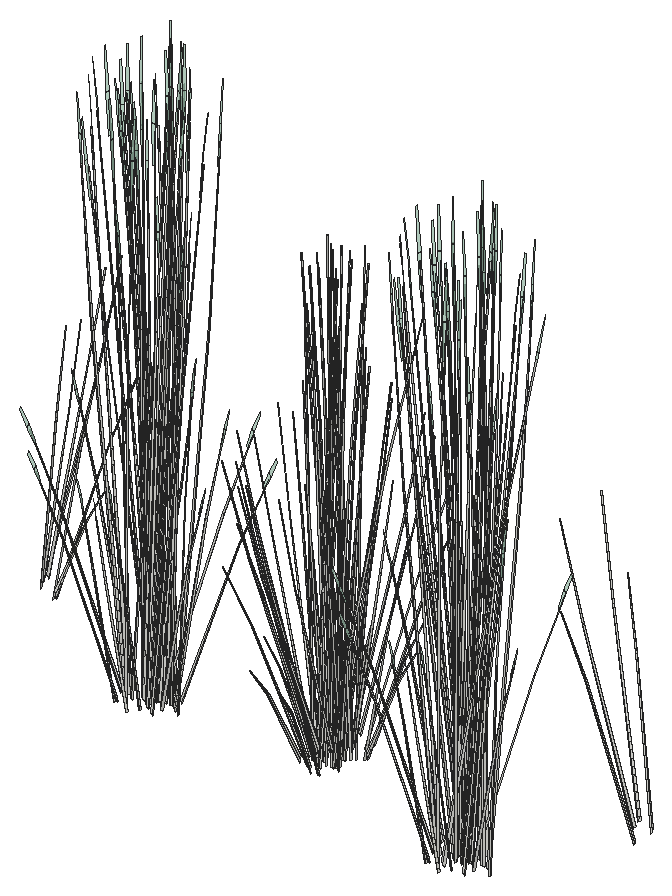
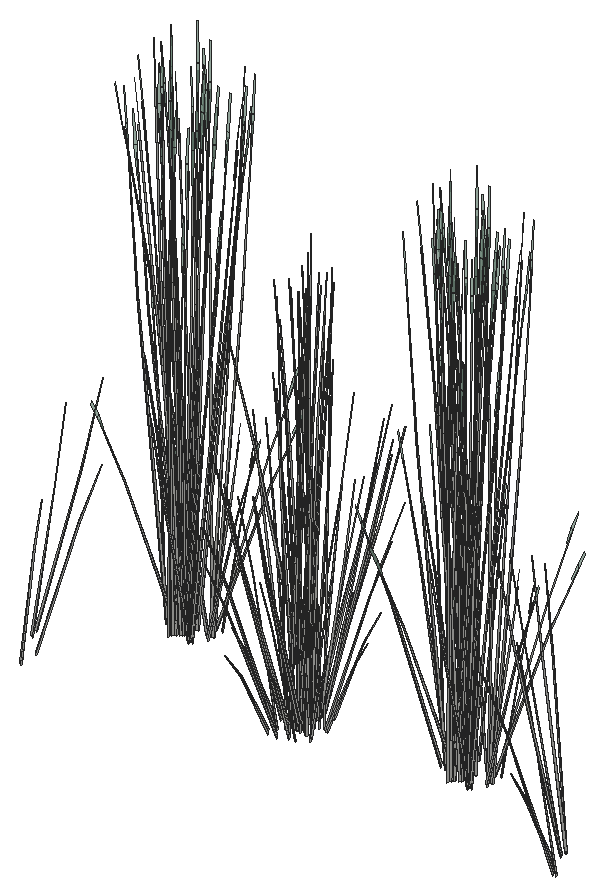
# SketchUp Ruby script. Lengths in inches.
U = 1.inch
M = Sketchup.active_model
def pt(a) = Geom::Point3d.new(a.map { |v| v * U })
def face(e, loops, mat)
  f = e.add_face(loops[0].map { |a| pt(a) })
  loops[1..].each { |l| e.add_face(l.map { |a| pt(a) }).erase! }
  f.material = f.back_material = mat if mat
  f
end
# faces: each face lists its corners as indices into pts; further lists are holes
def faces(e, pts, list, mat = nil) = list.each { |f| face(e, (f[0].is_a?(Array) ? f : [f]).map { |l| l.map { |i| pts[i] } }, mat) }
# xy, xz, yz: faces in a plane at the given z, y or x. An outline is a flat list of corners, or four numbers for a rectangle; further outlines are holes
def ring(l) = l.size == 4 ? [[l[0], l[1]], [l[2], l[1]], [l[2], l[3]], [l[0], l[3]]] : l.each_slice(2).to_a
def flat(e, list, mat, &to3) = list.each { |f| face(e, (f[0].is_a?(Array) ? f : [f]).map { |l| ring(l).map { |u, v| to3.(u, v) } }, mat) }
def xy(e, z, list, mat = nil) = flat(e, list, mat) { |x, y| [x, y, z] }
def xz(e, y, list, mat = nil) = flat(e, list, mat) { |x, z| [x, y, z] }
def yz(e, x, list, mat = nil) = flat(e, list, mat) { |y, z| [x, y, z] }
def lines(e, pts, list) = list.each { |a, b| e.add_line(pt(pts[a]), pt(pts[b])) }
# prism: a flat outline (further loops are holes) pulled along v
def prism(e, loops, v, mat = nil)
  f = face(e, loops, mat); d = Geom::Vector3d.new(v.map { |x| x * U })
  f.pushpull(f.normal.samedirection?(d) ? d.length : -d.length)
end
def box(e, o, s, mat = nil) = prism(e, [[o, [o[0] + s[0], o[1], o[2]], [o[0] + s[0], o[1] + s[1], o[2]], [o[0], o[1] + s[1], o[2]]]], [0, 0, s[2]], mat)
def at(x, y, z, deg = 0) = Geom::Transformation.translation(pt([x, y, z])) * Geom::Transformation.rotation(ORIGIN, Z_AXIS, deg.degrees)
def axes(o, x, y, z) = Geom::Transformation.new([*x, 0, *y, 0, *z, 0, *pt(o).to_a, 1])
def part(name) = M.definitions.add(name)
# library, detail: a bought-in or finely detailed component or shape, given as its bounding box
def library(name, o, s) = part(name).tap { |d| box(d.entities, o, s) }
def detail(e, o, s) = box(e.add_group.entities, o, s)
def put(e, d, t, mat = nil) = e.add_instance(d, t).tap { |i| i.material = mat if mat }
def group(e, t, mat = nil) = e.add_group.tap { |g| g.transformation = t; g.material = mat if mat }.entities
root = M.entities
M.materials.add("LightPink_Translucent").color = [175, 214, 192]
M.materials["LightPink_Translucent"].alpha = 0.75
c1 = part("blade")
p = [[2.15,0.21,22],[0,0.17,0],[0.09,0.45,0],[2.18,0.31,22],[2.29,0.31,22],[0.38,0.45,0],
  [2.48,0.24,33],[2.49,0.24,33],[2.48,0.22,33]]
faces(c1.entities,p,[[0,1,2,3],[4,5,2,3],[6,3,4,7],[8,0,3,6]])
c2 = part("blade with seeds\#1")
put(c2.entities,c1,at(0,0,0))
c3 = part("seeds")
p = [[0.3,-0.1,1.38],[-0.01,-0.03,1.59],[-0.01,-0.03,0.03],[0.14,-0.07,-0.07],[0.29,-0.03,3],[0.15,0.01,3.11]]
faces(c3.entities,p,[[0,1,2,3],[1,0,4,5]],"LightPink_Translucent")
c4 = part("blade with seeds")
put(c4.entities,c1,at(0,0,0))
put(c4.entities,c3,axes([2.4,0.25,30.99],[1.5799,-0.05474,1.17369],[-0.12525,1.92788,0.29478],[-0.07173,-0.02425,1.56792]))
put(root,c2,axes([413.42,244.55,138.99],[-0.22657,0.01287,0.94226],[0.1616,-0.32149,0.69231],[0.10799,0.06323,0.20754]))
put(root,c2,axes([412.55,244.43,140.82],[0.25603,-0.35588,-0.4653],[0.22422,0.37594,-0.36041],[0.13008,0.05415,0.89031]))
put(root,c2,axes([412.8,243.375,140.56],[0.09552,-0.48869,-0.41919],[0.3275,0.16751,-0.3247],[0.13186,-0.04481,0.80208]))
put(root,c2,axes([412.93,244.82,139.03],[-0.06748,-0.45162,0.05338],[0.27185,-0.10383,-0.708],[0.13761,0.02863,0.63462]))
put(root,c2,axes([412.43,244.54,141.1],[0.35246,0.01294,-0.64693],[-0.02367,0.54471,0.07807],[0.14932,0.05748,0.91515]))
put(root,c2,axes([412.73,243.55,140.8],[0.30983,-0.23727,-0.58282],[0.17267,0.48842,0.07033],[0.1497,-0.05548,0.82446]))
put(root,c2,axes([413.22,244.93,138.84],[-0.06011,-0.15688,1.17311],[0.18125,-0.38733,-0.25229],[0.15683,0.11528,0.50157]))
put(root,c4,axes([426.42,237.2,139.53],[0.1661,0.03656,1.30132],[0.10705,0.37341,-0.27986],[-0.22562,0.0699,0.55638]))
put(root,c4,axes([427.06,235.39,139.53],[0.09331,0.12399,1.30132],[-0.21502,0.33702,-0.27986],[-0.22079,-0.08055,0.55638]))
put(root,c4,axes([427.94,237.98,139.33],[-0.29882,0.44625,0],[-0.49993,-0.24886,-0.46963],[-0.11386,-0.05668,1.48977]))
put(root,c4,axes([427.4,238.63,139.53],[0.15082,-0.07025,1.30132],[0.37238,0.21183,-0.27986],[-0.11083,0.18329,0.55638]))
put(root,c4,axes([427.18,234.62,139.11],[-0.13787,0.36364,-0.03542],[-0.42434,-0.11186,-0.16061],[-0.06443,-0.05948,0.52975]))
put(root,c4,axes([427.82,234.16,139.53],[-0.02894,0.14568,1.30132],[-0.4231,0.12195,-0.27986],[-0.0989,-0.1883,0.55638]))
put(root,c4,axes([426.96,236.28,139.33],[-0.59763,0,0],[0,-0.49772,-0.46963],[0,-0.11336,1.48977]))
put(root,c4,axes([427.42,236.15,139.29],[-0.44456,0.37441,0.27988],[-0.44483,-0.37047,-0.33208],[-0.01552,-0.10632,1.50045]))
put(root,c4,axes([429.43,237.0625,139.41],[-0.4667,-0.35844,-0.22925],[0.39271,-0.40249,0.50168],[-0.12567,0.04193,1.53076]))
put(root,c4,axes([428.2,237.75,139.43],[0.44731,0.22267,0.45182],[-0.26736,0.39927,0],[-0.10188,-0.05071,1.43328]))
put(root,c4,axes([428.625,236.93,139.39],[0.12668,-0.5277,-0.2132],[0.60063,0.09198,0.46656],[-0.10495,-0.07287,1.42361]))
put(root,c4,axes([428.84,237.06,139.55],[-0.0922,0.39744,0.13176],[-0.45047,-0.06899,-0.37626],[-0.08198,-0.04081,1.15337]))
put(root,c4,axes([427.32,236.36,139.43],[0,0.44533,0.45182],[-0.53472,0,0],[0,-0.10143,1.43328]))
put(root,c4,axes([429.77,238.04,139.17],[-0.29509,-0.44781,-0.04679],[0.49993,-0.24886,0.46963],[-0.12319,0.04264,1.48904]))
put(root,c4,axes([427.5,238.29,139.74],[0.43418,-0.07886,0.05922],[0.09982,0.31771,-0.78537],[-0.02753,0.16083,0.70398]))
put(root,c4,axes([428.83,234.16,139.11],[-0.33028,0.25548,-0.03542],[-0.30262,-0.27981,-0.16061],[-0.02131,-0.07928,0.52975]))
put(root,c4,axes([428.69,236.68,139.32],[0.60408,0.09383,0.41637],[-0.12294,0.52992,0.16339],[-0.08828,-0.05117,1.44559]))
put(root,c4,axes([428.37,237.52,139.42],[0.51358,-0.1182,0.16054],[0.12682,0.43988,0.31929],[-0.0458,-0.06409,1.4597]))
put(root,c4,axes([429.03,237.59,139.17],[-0.48183,-0.19993,0],[0.23189,-0.41543,0],[0,0,1.48063]))
put(root,c4,axes([430.14,238.09,139.33],[0.29882,0.44625,0],[-0.49993,0.24886,-0.46963],[-0.11386,0.05668,1.48977]))
put(root,c4,axes([429.9,237.55,139.42],[0.13807,-0.44258,0.16054],[0.50524,0.12525,0.31929],[-0.08728,0.00216,1.4597]))
put(root,c4,axes([429.66,236.96,139.55],[0.3531,0.26757,0.13176],[-0.29453,0.30187,-0.37626],[-0.08198,0.04081,1.15337]))
put(root,c4,axes([429.54,236.63,139.26],[-0.44456,-0.3833,-0.05579],[0.44483,-0.38354,0],[-0.01552,-0.01339,1.5977]))
put(root,c4,axes([429.78,237.8125,139.29],[0.59835,0.14475,0.27988],[-0.14969,0.51739,-0.33208],[-0.09903,0.06475,1.50045]))
put(root,c4,axes([430.04,237.78,139.43],[0.44731,-0.22267,0.45182],[0.26736,0.39927,0],[-0.10188,0.05071,1.43328]))
put(root,c4,axes([428.64,236.1875,139.32],[0.2078,0.49797,0.41637],[-0.59373,0.17316,0.16339],[0.00726,-0.0915,1.44559]))
put(root,c4,axes([429.14,237.42,139.18],[-0.15594,-0.38394,0],[0.4453,-0.13445,0],[0,0,1.40478]))
put(root,c4,axes([430.69,236.42,139.42],[-0.37551,-0.32439,0.16054],[0.37842,-0.31463,0.31929],[-0.04147,0.06625,1.4597]))
put(root,c4,axes([429.39,236.23,139.18],[0,-0.51528,0],[0.59763,0,0],[0,0,1.63305]))
put(root,c4,axes([428.83,236.32,139.38],[0.53851,0.21584,0.21899],[-0.25917,0.44849,0.45502],[0,-0.10338,1.46094]))
put(root,c4,axes([429.6875,236.4375,139.26],[0,0.51503,-0.0513],[-0.59763,0,0],[0,0.01619,1.63225]))
put(root,c4,axes([428.42,235.24,139.42],[-0.13807,0.44258,0.16054],[-0.50524,-0.12525,0.31929],[0.08728,-0.00216,1.4597]))
put(root,c4,axes([429.4,237.43,139.25],[0.2078,0.51161,-0.05471],[-0.59373,0.17927,0],[0.00726,0.01787,1.56677]))
put(root,c4,axes([428.17,234.69,139.33],[-0.29882,-0.44625,0],[0.49993,-0.24886,-0.46963],[0.11386,-0.05668,1.48977]))
put(root,c4,axes([431.12,236.76,139.17],[-0.59734,-0.00356,-0.04529],[0,-0.49772,0.45448],[-0.01877,0.1133,1.441]))
put(root,c4,axes([429.95,235.26,139.42],[-0.51358,0.1182,0.16054],[-0.12682,-0.43988,0.31929],[0.0458,0.06409,1.4597]))
put(root,c4,axes([429.11,235.91,139.32],[-0.39628,0.40415,0.41637],[-0.4708,-0.35675,0.16339],[0.09554,-0.04033,1.44559]))
put(root,c4,axes([429.78,236.54,139.19],[0.33362,0.28765,0],[-0.33362,0.28765,0],[0,0,1.54032]))
put(root,c4,axes([429.58,237.6,139.18],[0.48183,0.19993,0],[-0.23189,0.41543,0],[0,0,1.59208]))
put(root,c4,axes([429.62,236.11,139.34],[-0.60408,-0.09383,0.44771],[0.12294,-0.52992,0.17569],[0.08828,0.05117,1.5544]))
put(root,c4,axes([429.79,236.35,139.18],[0.53472,0,0],[0,0.46104,0],[0,0,1.6235]))
put(root,c4,axes([429.98,236.3,139.55],[0.4453,-0.12987,0.13176],[0.15594,0.37086,-0.37626],[0,0.08162,1.15337]))
put(root,c4,axes([429.92,234.33,139.53],[-0.13585,0.09014,1.30132],[-0.40687,-0.15777,-0.27986],[0.07542,-0.19621,0.55638]))
put(root,c4,axes([430.99,236.43,139.43],[0,-0.44533,0.45182],[0.53472,0,0],[0,0.10143,1.43328]))
put(root,c4,axes([429.47,235.73,139.55],[0.0922,-0.39744,0.13176],[0.45047,0.06899,-0.37626],[0.08198,0.04081,1.15337]))
put(root,c4,axes([430.11,235.04,139.43],[-0.44731,-0.22267,0.45182],[0.26736,-0.39927,0],[0.10188,0.05071,1.43328]))
put(root,c4,axes([429.72,237.37,139.16],[0.50177,-0.1511,-0.1747],[0.17632,0.43526,0.00007],[0.05539,-0.0167,1.58246]))
put(root,c4,axes([429.59,237.63,139.53],[0.00843,-0.14762,1.30132],[0.40305,-0.1649,-0.27986],[0.12442,0.17669,0.55638]))
put(root,c4,axes([431.36,236.51,139.33],[0.59763,0,0],[0,0.49772,-0.46963],[0,0.11336,1.48977]))
put(root,c4,axes([430.37,234.81,139.33],[0.29882,-0.44625,0],[0.49993,0.24886,-0.46963],[0.11386,0.05668,1.48977]))
put(root,c4,axes([432.11,236.19,139.23],[-0.29631,-0.28477,-0.05904],[0.32453,-0.26092,-0.26768],[0.09195,-0.01837,0.88292]))
put(root,c4,axes([431.23,235.39,139.53],[-0.17074,-0.01319,1.30132],[-0.17492,-0.35385,-0.27986],[0.20976,-0.1001,0.55638]))
put(root,c4,axes([431.55,236.57,138.97],[-0.30783,0.05344,1.28841],[-0.049,-0.4254,0.07375],[0.2156,-0.06439,0.73315]))
put(root,c4,axes([431.63,237.2,139.53],[-0.1151,-0.10953,1.30132],[0.14976,-0.36232,-0.27986],[0.23288,0.04908,0.55638]))
put(root,c2,axes([443.83,237.48,138.9375],[0.07713,0.14131,1.17311],[-0.13499,0.4232,-0.25229],[-0.16789,-0.07845,0.50157]))
put(root,c2,axes([444.1,238.13,140.9],[-0.30983,0.23727,-0.58282],[-0.17267,-0.48842,0.07033],[-0.1497,0.05548,0.82446]))
put(root,c2,axes([443.6875,239.67,138.9375],[0.12465,0.0301,1.17311],[0.10435,0.44009,-0.25229],[-0.16111,0.10287,0.50157]))
put(root,c2,axes([444.41,237.14,140.9],[-0.35246,-0.01294,-0.58282],[0.02367,-0.54471,0.07033],[-0.14932,-0.05748,0.82446]))
put(root,c2,axes([443.22,238.01,139.08],[0.2222,-0.06377,0.94226],[-0.12306,0.35378,0.69231],[-0.11377,-0.03807,0.20754]))
put(root,c2,axes([444.04,238.31,140.65],[-0.09552,0.48869,-0.41919],[-0.3275,-0.16751,-0.3247],[-0.13186,0.04481,0.80208]))
put(root,c2,axes([444.29,237.25,140.65],[-0.25603,0.35588,-0.41919],[-0.22422,-0.37594,-0.3247],[-0.13008,-0.05415,0.80208]))
put(root,c2,axes([443.49,239.82,139.08],[0.13262,-0.25932,0.94226],[0.07972,0.37767,0.69231],[-0.10192,0.08081,0.20754]))
put(root,c2,axes([444.19,239.2,140.9],[-0.18418,0.4239,-0.58282],[-0.32274,-0.30126,0.07033],[-0.10997,0.15358,0.82446]))
put(root,c2,axes([444.2,239.4,140.65],[0.09058,0.49056,-0.41919],[-0.34303,0.08581,-0.3247],[-0.0983,0.13176,0.80208]))
put(root,c2,axes([444.88,236.51,140.65],[-0.34793,0.12771,-0.41919],[-0.06086,-0.48364,-0.3247],[-0.09345,-0.1386,0.80208]))
put(root,c2,axes([445.02,236.5,140.9],[-0.30066,-0.25968,-0.58282],[0.21367,-0.45504,0.07033],[-0.10893,-0.15505,0.82446]))
put(root,c2,axes([444.74,236.125,138.9375],[-0.01129,0.1776,1.17311],[-0.30276,0.18194,-0.25229],[-0.08565,-0.21818,0.50157]))
put(root,c2,axes([444.1875,235.92,139.08],[0.19397,0.16559,0.94226],[-0.26061,0.14233,0.69231],[-0.0653,-0.13676,0.20754]))
put(root,c2,axes([444.74,240.46,138.9375],[0.10609,-0.09706,1.17311],[0.28837,0.22366,-0.25229],[-0.06892,0.22965,0.50157]))
put(root,c2,axes([444.65,240.0625,140.9],[-0.00917,0.49695,-0.58282],[-0.38634,-0.03338,0.07033],[-0.04077,0.21053,0.82446]))
put(root,c2,axes([444.72,240.23,140.65],[0.25241,0.36098,-0.41919],[-0.26664,0.31614,-0.3247],[-0.0384,0.18341,0.80208]))
put(root,c2,axes([445.54,238.62,138.81],[0.18468,-0.56014,0.19741],[0.38374,0.26958,0.41019],[-0.08846,0,1.31701]))
put(root,c2,axes([445.06,241.04,139.08],[-0.02727,-0.31739,0.94226],[0.24024,0.20133,0.69231],[-0.03604,0.15684,0.20754]))
put(root,c2,axes([445.28,238.8,139.04],[0.02352,0.53984,0.36702],[-0.39046,0.04882,-0.17663],[-0.03957,-0.09664,1.17838]))
put(root,c2,axes([445.57,240.19,138.85],[0.38104,0,0.40731],[0,0.5562,0],[-0.08679,0,1.29208]))
put(root,c2,axes([445.42,238.82,138.75],[0.42608,-0.21614,0.37535],[0.14817,0.61757,0.14729],[-0.07829,-0.00755,1.30318]))
put(root,c2,axes([445.65,236.29,140.65],[-0.34661,-0.13468,-0.41919],[0.1188,-0.46175,-0.3247],[-0.03178,-0.18591,0.80208]))
put(root,c2,axes([444.4375,237.29,138.85],[-0.19052,0.46527,0.40731],[-0.34163,-0.2781,0],[0.04339,-0.10597,1.29208]))
put(root,c2,axes([445.76,238.93,139.04],[0.34335,0.2412,0.36702],[-0.16524,0.50118,-0.17663],[-0.07915,0,1.17838]))
put(root,c2,axes([445.18,238.33,138.75],[0.3458,0.41219,0.37535],[-0.30525,0.4897,0.14729],[-0.03451,-0.09937,1.30318]))
put(root,c2,axes([444.61,239.05,138.84],[0.37869,0.14361,0.14473],[-0.10717,0.52552,0.28783],[-0.00184,-0.09078,1.3159]))
put(root,c2,axes([445.78,236.375,140.9],[-0.16829,-0.43684,-0.58282],[0.34641,-0.24345,0.07033],[-0.03935,-0.21107,0.82446]))
put(root,c2,axes([445.03,237.95,138.96],[-0.34006,-0.0959,0.11878],[0.05903,-0.46856,-0.33919],[0.03492,-0.08527,1.03975]))
put(root,c2,axes([445.12,238.15,139.04],[-0.31983,0.29864,0.36702],[-0.22522,-0.45236,-0.17663],[0.03957,-0.09664,1.17838]))
put(root,c2,axes([445.84,238.76,138.75],[0.08028,-0.62833,0.37535],[0.45342,0.12787,0.14729],[-0.04378,0.09182,1.30318]))
put(root,c2,axes([444.63,237.46,138.84],[0.10113,0.5342,0.14473],[-0.37638,0.13191,0.28783],[0.05484,-0.04764,1.3159]))
put(root,c2,axes([446.5625,239.1,138.84],[-0.10113,-0.5342,0.14473],[0.37638,-0.13191,0.28783],[-0.05484,0.04764,1.3159]))
put(root,c2,axes([445.36,237.8,138.77],[-0.08028,0.62833,0.4036],[-0.45342,-0.12787,0.15838],[0.04378,-0.09182,1.40127]))
put(root,c2,axes([446.16,238.61,138.96],[0.34006,0.0959,0.11878],[-0.05903,0.46856,-0.33919],[-0.03492,0.08527,1.03975]))
put(root,c2,axes([445.73,237.63,138.63],[0.24613,-0.34702,0],[0.24613,0.34702,0],[0,0,1.38858]))
put(root,c2,axes([445.62,236.69,138.84],[-0.27756,0.39059,0.14473],[-0.26921,-0.39362,0.28783],[0.05668,0.04314,1.3159]))
put(root,c2,axes([445.87,235.13,139.08],[0.06291,0.30716,0.94226],[-0.25998,-0.14458,0.69231],[0.01779,-0.16295,0.20754]))
put(root,c2,axes([446.58,237.51,138.84],[-0.37869,-0.14361,0.14473],[0.10717,-0.52552,0.28783],[0.00184,0.09078,1.3159]))
put(root,c2,axes([445.4375,237.63,139.04],[-0.34335,-0.2412,0.36702],[0.16524,-0.50118,-0.17663],[0.07915,0,1.17838]))
put(root,c2,axes([446.76,239.27,138.85],[0.19052,-0.46527,0.40731],[0.34163,0.2781,0],[-0.04339,0.10597,1.29208]))
put(root,c2,axes([445.47,240.58,140.65],[0.34661,0.13468,-0.41919],[-0.1188,0.46175,-0.3247],[0.03178,0.18591,0.80208]))
put(root,c2,axes([445.63,236.37,138.85],[-0.38104,0,0.40731],[0,-0.5562,0],[0.08679,0,1.29208]))
put(root,c2,axes([445.52,237.42,138.96],[-0.11112,-0.46318,0.11878],[0.31732,-0.1622,-0.33919],[0.06984,0,1.03975]))
put(root,c2,axes([445.91,237.76,139.04],[-0.02352,-0.53984,0.36702],[0.39046,-0.04882,-0.17663],[0.03957,0.09664,1.17838]))
put(root,c2,axes([446.29,235.7,138.9375],[-0.09372,0.11973,1.17311],[-0.31002,-0.15578,-0.25229],[0.042,-0.24224,0.50157]))
put(root,c2,axes([446.08,237.75,138.96],[0.22894,-0.36728,0.11878],[0.25829,0.30636,-0.33919],[0.03492,0.08527,1.03975]))
put(root,c2,axes([446.48,236.8,140.9],[0.00917,-0.49695,-0.58282],[0.38634,0.03338,0.07033],[0.04077,-0.21053,0.82446]))
put(root,c2,axes([446.79,237.36,138.85],[-0.19052,-0.46527,0.40731],[0.34163,-0.2781,0],[0.04339,0.10597,1.29208]))
put(root,c2,axes([446.29,241.13,138.9375],[0.03128,-0.17277,1.17311],[0.3195,-0.11135,-0.25229],[0.05981,0.23468,0.50157]))
put(root,c2,axes([446.96,241.49,139.08],[-0.1727,-0.20718,0.94226],[0.27339,-0.08175,0.69231],[0.04895,0.14972,0.20754]))
put(root,c2,axes([446.77,236.84,139.08],[-0.10956,0.27991,0.94226],[-0.11132,-0.36143,0.69231],[0.0943,-0.09749,0.20754]))
put(root,c2,axes([446.25,240.35,140.65],[0.34793,-0.12771,-0.41919],[0.06086,0.48364,-0.3247],[0.09345,0.1386,0.80208]))
put(root,c2,axes([445.54,237.52,139.14],[-0.35877,0.01358,1.15892],[0.093,-0.61462,0.4907],[0.19631,0.14537,1.09393]))
put(root,c2,axes([446.92,237.47,140.65],[-0.09058,-0.49056,-0.41919],[0.34303,-0.08581,-0.3247],[0.0983,-0.13176,0.80208]))
put(root,c2,axes([447.27,236.79,139],[-0.01195,0.31879,0.86186],[-0.25381,-0.21053,0.47585],[0.09017,-0.12594,0.67605]))
put(root,c2,axes([446.66,237.83,138.9375],[-0.12631,-0.00877,1.17311],[-0.14109,-0.41923,-0.25229],[0.15118,-0.12942,0.50157]))
put(root,c2,axes([447.71,239.73,139.08],[-0.22657,0.01287,0.94226],[0.1616,-0.32149,0.69231],[0.10799,0.06323,0.20754]))
put(root,c2,axes([447.08,238.56,140.65],[0.09552,-0.48869,-0.41919],[0.3275,0.16751,-0.3247],[0.13186,-0.04481,0.80208]))
put(root,c2,axes([447.22,240,139.13],[-0.06748,-0.45162,0.05338],[0.27185,-0.10383,-0.708],[0.13761,0.02863,0.63462]))
put(root,c2,axes([447.02,238.74,140.9],[0.30983,-0.23727,-0.58282],[0.17267,0.48842,0.07033],[0.1497,-0.05548,0.82446]))
put(root,c2,axes([447.51,240.11,138.9375],[-0.06011,-0.15688,1.17311],[0.18125,-0.38733,-0.25229],[0.15683,0.11528,0.50157]))
put(root,c4,axes([460.7,232.38,139.62],[0.1661,0.03656,1.30132],[0.10705,0.37341,-0.27986],[-0.22562,0.0699,0.55638]))
put(root,c4,axes([461.35,230.57,139.62],[0.09331,0.12399,1.30132],[-0.21502,0.33702,-0.27986],[-0.22079,-0.08055,0.55638]))
put(root,c4,axes([462.23,233.16,139.42],[-0.29882,0.44625,0],[-0.49993,-0.24886,-0.46963],[-0.11386,-0.05668,1.48977]))
put(root,c4,axes([461.6875,233.81,139.62],[0.15082,-0.07025,1.30132],[0.37238,0.21183,-0.27986],[-0.11083,0.18329,0.55638]))
put(root,c4,axes([461.47,229.8,139.2],[-0.13787,0.36364,-0.03542],[-0.42434,-0.11186,-0.16061],[-0.06443,-0.05948,0.52975]))
put(root,c4,axes([462.11,229.35,139.62],[-0.02894,0.14568,1.30132],[-0.4231,0.12195,-0.27986],[-0.0989,-0.1883,0.55638]))
put(root,c4,axes([463.18,232.11,139.69],[-0.48255,0.29566,-0.26477],[-0.32089,-0.41776,-0.45502],[-0.11906,-0.04243,1.45334]))
put(root,c4,axes([461.24,231.46,139.42],[-0.59763,0,0],[0,-0.49772,-0.46963],[0,-0.11336,1.48977]))
put(root,c4,axes([461.71,231.33,139.39],[-0.44456,0.37441,0.27988],[-0.44483,-0.37047,-0.33208],[-0.01552,-0.10632,1.50045]))
put(root,c4,axes([463.72,232.24,139.51],[-0.4667,-0.35844,-0.22925],[0.39271,-0.40249,0.50168],[-0.12567,0.04193,1.53076]))
put(root,c4,axes([462.91,232.11,139.48],[0.12668,-0.5277,-0.2132],[0.60063,0.09198,0.46656],[-0.10495,-0.07287,1.42361]))
put(root,c4,axes([463.13,232.24,139.65],[-0.0922,0.39744,0.13176],[-0.45047,-0.06899,-0.37626],[-0.08198,-0.04081,1.15337]))
put(root,c4,axes([464.06,233.23,139.26],[-0.29509,-0.44781,-0.04679],[0.49993,-0.24886,0.46963],[-0.12319,0.04264,1.48904]))
put(root,c4,axes([462.78,231.64,139.69],[-0.53825,-0.21249,-0.26477],[0.25917,-0.44849,-0.45502],[-0.01692,-0.11011,1.45334]))
put(root,c4,axes([461.79,233.47,139.83],[0.43418,-0.07886,0.05922],[0.09982,0.31771,-0.78537],[-0.02753,0.16083,0.70398]))
put(root,c4,axes([463.84,232.04,139.69],[0.05569,0.50815,-0.26477],[-0.58006,0.03072,-0.45502],[-0.10214,0.06769,1.45334]))
put(root,c4,axes([463.11,229.34,139.2],[-0.33028,0.25548,-0.03542],[-0.30262,-0.27981,-0.16061],[-0.02131,-0.07928,0.52975]))
put(root,c4,axes([462.98,231.86,139.41],[0.60408,0.09383,0.41637],[-0.12294,0.52992,0.16339],[-0.08828,-0.05117,1.44559]))
put(root,c4,axes([463.32,232.78,139.26],[-0.48183,-0.19993,0],[0.23189,-0.41543,0],[0,0,1.48063]))
put(root,c4,axes([464.43,233.28,139.42],[0.29882,0.44625,0],[-0.49993,0.24886,-0.46963],[-0.11386,0.05668,1.48977]))
put(root,c4,axes([463.95,232.14,139.65],[0.3531,0.26757,0.13176],[-0.29453,0.30187,-0.37626],[-0.08198,0.04081,1.15337]))
put(root,c4,axes([463.83,231.8125,139.36],[-0.44456,-0.3833,-0.05579],[0.44483,-0.38354,0],[-0.01552,-0.01339,1.5977]))
put(root,c4,axes([464.07,233,139.39],[0.59835,0.14475,0.27988],[-0.14969,0.51739,-0.33208],[-0.09903,0.06475,1.50045]))
put(root,c4,axes([462.93,231.37,139.41],[0.2078,0.49797,0.41637],[-0.59373,0.17316,0.16339],[0.00726,-0.0915,1.44559]))
put(root,c4,axes([463.43,232.6,139.27],[-0.15594,-0.38394,0],[0.4453,-0.13445,0],[0,0,1.40478]))
put(root,c4,axes([463.68,231.41,139.27],[0,-0.51528,0],[0.59763,0,0],[0,0,1.63305]))
put(root,c4,axes([463.12,231.51,139.48],[0.53851,0.21584,0.21899],[-0.25917,0.44849,0.45502],[0,-0.10338,1.46094]))
put(root,c4,axes([463.98,231.62,139.35],[0,0.51503,-0.0513],[-0.59763,0,0],[0,0.01619,1.63225]))
put(root,c4,axes([463.69,232.62,139.35],[0.2078,0.51161,-0.05471],[-0.59373,0.17927,0],[0.00726,0.01787,1.56677]))
put(root,c4,axes([462.46,229.875,139.42],[-0.29882,-0.44625,0],[0.49993,-0.24886,-0.46963],[0.11386,-0.05668,1.48977]))
put(root,c4,axes([465.41,231.94,139.27],[-0.59734,-0.00356,-0.04529],[0,-0.49772,0.45448],[-0.01877,0.1133,1.441]))
put(root,c4,axes([463.39,231.09,139.41],[-0.39628,0.40415,0.41637],[-0.4708,-0.35675,0.16339],[0.09554,-0.04033,1.44559]))
put(root,c4,axes([464.07,231.73,139.28],[0.33362,0.28765,0],[-0.33362,0.28765,0],[0,0,1.54032]))
put(root,c4,axes([463.86,232.78,139.27],[0.48183,0.19993,0],[-0.23189,0.41543,0],[0,0,1.59208]))
put(root,c4,axes([463.91,231.29,139.43],[-0.60408,-0.09383,0.44771],[0.12294,-0.52992,0.17569],[0.08828,0.05117,1.5544]))
put(root,c4,axes([464.08,231.53,139.27],[0.53472,0,0],[0,0.46104,0],[0,0,1.6235]))
put(root,c4,axes([463.04,231.11,139.69],[-0.05569,-0.50815,-0.26477],[0.58006,-0.03072,-0.45502],[0.10214,-0.06769,1.45334]))
put(root,c4,axes([464.27,231.48,139.65],[0.4453,-0.12987,0.13176],[0.15594,0.37086,-0.37626],[0,0.08162,1.15337]))
put(root,c4,axes([464.11,231.51,139.69],[0.53825,0.21249,-0.26477],[-0.25917,0.44849,-0.45502],[0.01692,0.11011,1.45334]))
put(root,c4,axes([464.21,229.52,139.62],[-0.13585,0.09014,1.30132],[-0.40687,-0.15777,-0.27986],[0.07542,-0.19621,0.55638]))
put(root,c4,axes([463.76,230.91,139.65],[0.0922,-0.39744,0.13176],[0.45047,0.06899,-0.37626],[0.08198,0.04081,1.15337]))
put(root,c4,axes([464.01,232.55,139.25],[0.50177,-0.1511,-0.1747],[0.17632,0.43526,0.00007],[0.05539,-0.0167,1.58246]))
put(root,c4,axes([463.875,232.8125,139.62],[0.00843,-0.14762,1.30132],[0.40305,-0.1649,-0.27986],[0.12442,0.17669,0.55638]))
put(root,c4,axes([465.65,231.6875,139.43],[0.59763,0,0],[0,0.49772,-0.46963],[0,0.11336,1.48977]))
put(root,c4,axes([463.71,231.04,139.69],[0.48255,-0.29566,-0.26477],[0.32089,0.41776,-0.45502],[0.11906,0.04243,1.45334]))
put(root,c4,axes([462.5,230.78,138.72],[-0.47044,0.17829,1.17325],[-0.14973,-0.51157,0.45588],[0.28888,0.00851,1.33444]))
put(root,c4,axes([464.66,229.99,139.43],[0.29882,-0.44625,0],[0.49993,0.24886,-0.46963],[0.11386,0.05668,1.48977]))
put(root,c4,axes([466.39,231.375,139.32],[-0.29631,-0.28477,-0.05904],[0.32453,-0.26092,-0.26768],[0.09195,-0.01837,0.88292]))
put(root,c2,axes([471.56,242.3,138.84],[0.07713,0.14131,1.17311],[-0.13499,0.4232,-0.25229],[-0.16789,-0.07845,0.50157]))
put(root,c2,axes([471.83,242.95,140.8],[-0.30983,0.23727,-0.58282],[-0.17267,-0.48842,0.07033],[-0.1497,0.05548,0.82446]))
put(root,c2,axes([471.41,244.49,138.84],[0.12465,0.0301,1.17311],[0.10435,0.44009,-0.25229],[-0.16111,0.10287,0.50157]))
put(root,c4,axes([465.52,230.58,139.62],[-0.17074,-0.01319,1.30132],[-0.17492,-0.35385,-0.27986],[0.20976,-0.1001,0.55638]))
put(root,c2,axes([472.13,241.96,140.8],[-0.35246,-0.01294,-0.58282],[0.02367,-0.54471,0.07033],[-0.14932,-0.05748,0.82446]))
